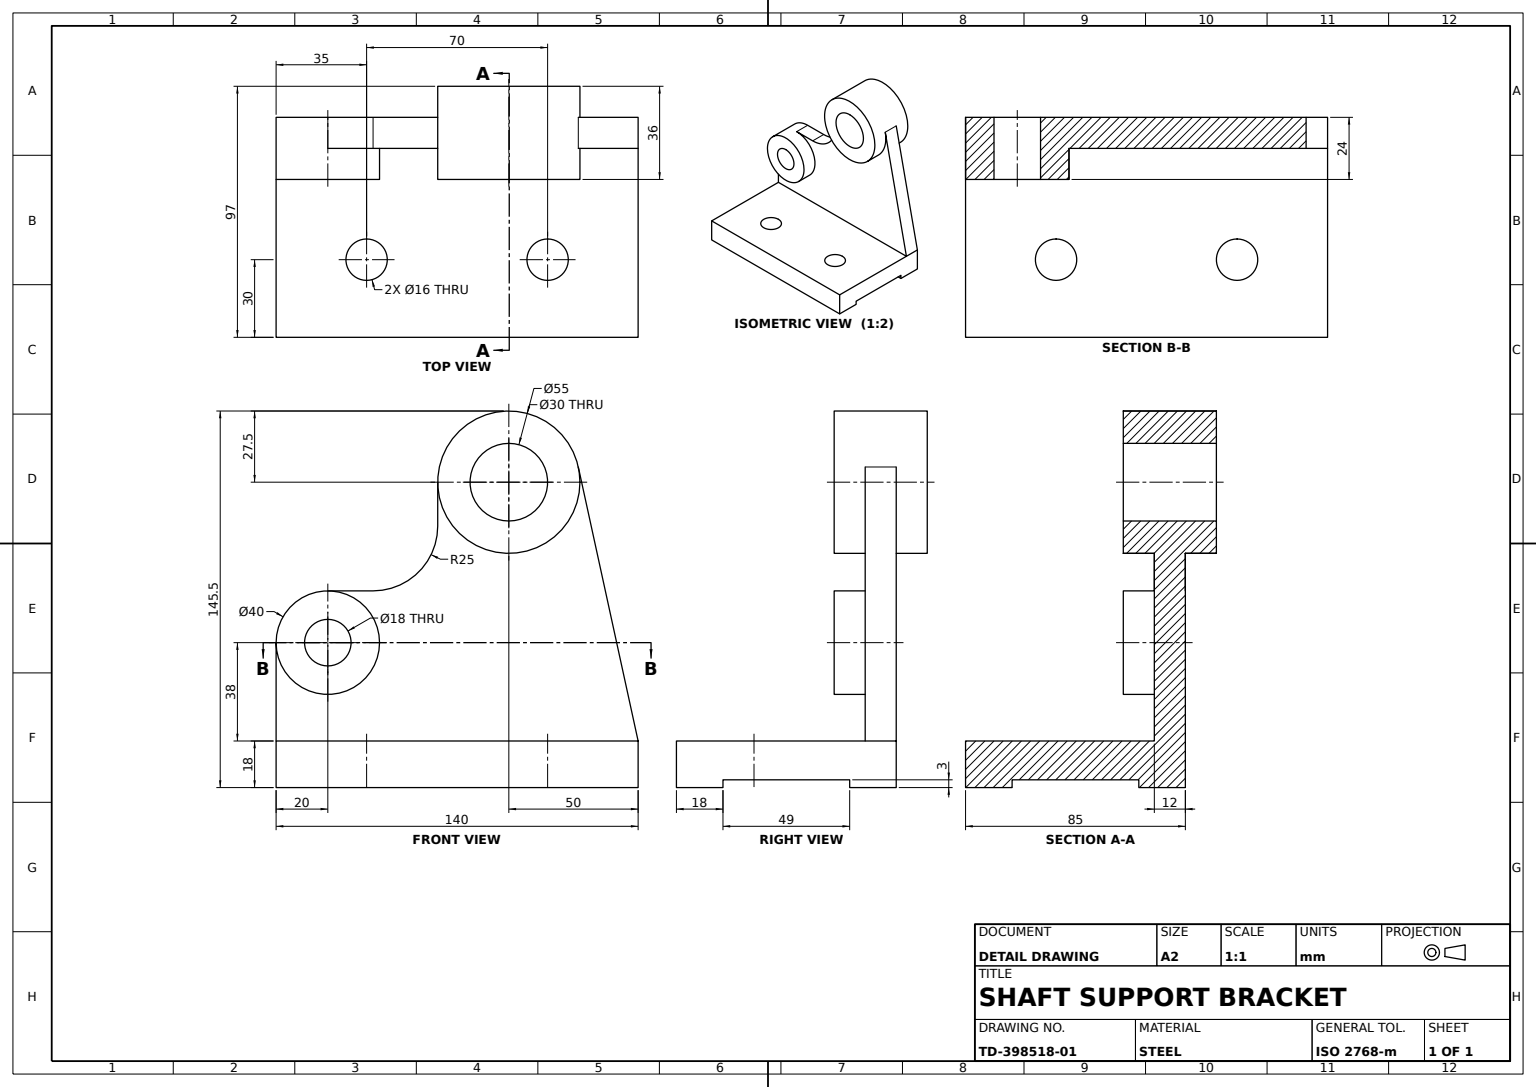
ISO-10303-21;
HEADER;
FILE_DESCRIPTION((''),'2;1');
FILE_NAME('','',(''),(''),'','','');
FILE_SCHEMA(('AUTOMOTIVE_DESIGN'));
ENDSEC;
DATA;
#1=APPLICATION_CONTEXT('');
#2=PRODUCT_CONTEXT('',#1,'mechanical');
#3=PRODUCT('','','',(#2));
#4=PRODUCT_DEFINITION_FORMATION('','',#3);
#5=PRODUCT_DEFINITION_CONTEXT('',#1,'design');
#6=PRODUCT_DEFINITION('','',#4,#5);
#7=PRODUCT_DEFINITION_SHAPE('','',#6);
#8=(LENGTH_UNIT()NAMED_UNIT(*)SI_UNIT(.MILLI.,.METRE.));
#9=(NAMED_UNIT(*)PLANE_ANGLE_UNIT()SI_UNIT($,.RADIAN.));
#10=(NAMED_UNIT(*)SI_UNIT($,.STERADIAN.)SOLID_ANGLE_UNIT());
#11=UNCERTAINTY_MEASURE_WITH_UNIT(LENGTH_MEASURE(0.005),#8,'distance_accuracy_value','');
#12=(GEOMETRIC_REPRESENTATION_CONTEXT(3)GLOBAL_UNCERTAINTY_ASSIGNED_CONTEXT((#11))GLOBAL_UNIT_ASSIGNED_CONTEXT((#8,#9,#10))REPRESENTATION_CONTEXT('',''));
#13=CARTESIAN_POINT('',(-18.5,-50.,65.));
#14=VERTEX_POINT('',#13);
#15=CARTESIAN_POINT('',(-18.5,-50.,56.));
#16=DIRECTION('',(-1.,0.,0.));
#17=DIRECTION('',(0.,0.,1.));
#18=AXIS2_PLACEMENT_3D('',#15,#16,#17);
#19=CIRCLE('',#18,9.);
#20=EDGE_CURVE('',#14,#14,#19,.T.);
#21=ORIENTED_EDGE('',*,*,#20,.T.);
#22=EDGE_LOOP('',(#21));
#23=FACE_BOUND('',#22,.T.);
#24=CARTESIAN_POINT('',(-18.5,-30.,56.));
#25=VERTEX_POINT('',#24);
#26=DIRECTION('',(1.,0.,0.));
#27=DIRECTION('',(0.,1.,0.));
#28=AXIS2_PLACEMENT_3D('',#15,#26,#27);
#29=CIRCLE('',#28,20.);
#30=EDGE_CURVE('',#25,#25,#29,.T.);
#31=ORIENTED_EDGE('',*,*,#30,.T.);
#32=EDGE_LOOP('',(#31));
#33=FACE_BOUND('',#32,.T.);
#34=DIRECTION('',(0.,0.,-1.));
#35=AXIS2_PLACEMENT_3D('',#15,#26,#34);
#36=PLANE('',#35);
#37=ADVANCED_FACE('',(#23,#33),#36,.T.);
#38=CARTESIAN_POINT('',(20.5,35.,3.));
#39=VERTEX_POINT('',#38);
#40=CARTESIAN_POINT('',(12.5,35.,3.));
#41=AXIS2_PLACEMENT_3D('',#40,#17,#26);
#42=CIRCLE('',#41,8.);
#43=EDGE_CURVE('',#39,#39,#42,.T.);
#44=ORIENTED_EDGE('',*,*,#43,.T.);
#45=EDGE_LOOP('',(#44));
#46=FACE_BOUND('',#45,.T.);
#47=CARTESIAN_POINT('',(20.5,-35.,3.));
#48=VERTEX_POINT('',#47);
#49=CARTESIAN_POINT('',(12.5,-35.,3.));
#50=AXIS2_PLACEMENT_3D('',#49,#17,#26);
#51=CIRCLE('',#50,8.);
#52=EDGE_CURVE('',#48,#48,#51,.T.);
#53=ORIENTED_EDGE('',*,*,#52,.T.);
#54=EDGE_LOOP('',(#53));
#55=FACE_BOUND('',#54,.T.);
#56=CARTESIAN_POINT('',(-24.5,-70.,3.));
#57=VERTEX_POINT('',#56);
#58=CARTESIAN_POINT('',(24.5,-70.,3.));
#59=VERTEX_POINT('',#58);
#60=CARTESIAN_POINT('',(0.,-70.,3.));
#61=VECTOR('',#26,1000.);
#62=LINE('',#60,#61);
#63=EDGE_CURVE('',#57,#59,#62,.T.);
#64=ORIENTED_EDGE('',*,*,#63,.F.);
#65=CARTESIAN_POINT('',(-24.5,70.,3.));
#66=VERTEX_POINT('',#65);
#67=CARTESIAN_POINT('',(-24.5,-78.,3.));
#68=VECTOR('',#27,1000.);
#69=LINE('',#67,#68);
#70=EDGE_CURVE('',#66,#57,#69,.F.);
#71=ORIENTED_EDGE('',*,*,#70,.F.);
#72=CARTESIAN_POINT('',(24.5,70.,3.));
#73=VERTEX_POINT('',#72);
#74=CARTESIAN_POINT('',(0.,70.,3.));
#75=LINE('',#74,#61);
#76=EDGE_CURVE('',#66,#73,#75,.T.);
#77=ORIENTED_EDGE('',*,*,#76,.T.);
#78=CARTESIAN_POINT('',(24.5,-78.,3.));
#79=LINE('',#78,#68);
#80=EDGE_CURVE('',#73,#59,#79,.F.);
#81=ORIENTED_EDGE('',*,*,#80,.T.);
#82=EDGE_LOOP('',(#64,#71,#77,#81));
#83=FACE_BOUND('',#82,.T.);
#84=AXIS2_PLACEMENT_3D('',#67,#17,#26);
#85=PLANE('',#84);
#86=ADVANCED_FACE('',(#46,#55,#83),#85,.F.);
#87=ORIENTED_EDGE('',*,*,#30,.F.);
#88=EDGE_LOOP('',(#87));
#89=FACE_BOUND('',#88,.T.);
#90=CARTESIAN_POINT('',(-42.5,-70.,56.));
#91=VERTEX_POINT('',#90);
#92=CARTESIAN_POINT('',(-30.5,-70.,56.));
#93=VERTEX_POINT('',#92);
#94=LINE('',#90,#61);
#95=EDGE_CURVE('',#91,#93,#94,.T.);
#96=ORIENTED_EDGE('',*,*,#95,.T.);
#97=CARTESIAN_POINT('',(-30.5,-50.,76.));
#98=VERTEX_POINT('',#97);
#99=CARTESIAN_POINT('',(-30.5,-50.,56.));
#100=AXIS2_PLACEMENT_3D('',#99,#16,#17);
#101=CIRCLE('',#100,20.);
#102=EDGE_CURVE('',#93,#98,#101,.F.);
#103=ORIENTED_EDGE('',*,*,#102,.T.);
#104=CARTESIAN_POINT('',(-42.5,-50.,76.));
#105=VERTEX_POINT('',#104);
#106=LINE('',#104,#61);
#107=EDGE_CURVE('',#105,#98,#106,.T.);
#108=ORIENTED_EDGE('',*,*,#107,.F.);
#109=CARTESIAN_POINT('',(-42.5,-50.,56.));
#110=AXIS2_PLACEMENT_3D('',#109,#16,#27);
#111=CIRCLE('',#110,20.);
#112=EDGE_CURVE('',#91,#105,#111,.T.);
#113=ORIENTED_EDGE('',*,*,#112,.F.);
#114=EDGE_LOOP('',(#96,#103,#108,#113));
#115=FACE_BOUND('',#114,.T.);
#116=AXIS2_PLACEMENT_3D('',#109,#26,#34);
#117=CYLINDRICAL_SURFACE('',#116,20.);
#118=ADVANCED_FACE('',(#89,#115),#117,.T.);
#119=CARTESIAN_POINT('',(4.5,35.,18.));
#120=VERTEX_POINT('',#119);
#121=CARTESIAN_POINT('',(12.5,35.,18.));
#122=AXIS2_PLACEMENT_3D('',#121,#34,#16);
#123=CIRCLE('',#122,8.);
#124=EDGE_CURVE('',#120,#120,#123,.T.);
#125=ORIENTED_EDGE('',*,*,#124,.T.);
#126=EDGE_LOOP('',(#125));
#127=FACE_BOUND('',#126,.T.);
#128=CARTESIAN_POINT('',(42.5,70.,18.));
#129=VERTEX_POINT('',#128);
#130=CARTESIAN_POINT('',(42.5,-70.,18.));
#131=VERTEX_POINT('',#130);
#132=DIRECTION('',(0.,-1.,0.));
#133=VECTOR('',#132,1000.);
#134=LINE('',#128,#133);
#135=EDGE_CURVE('',#129,#131,#134,.T.);
#136=ORIENTED_EDGE('',*,*,#135,.F.);
#137=CARTESIAN_POINT('',(-30.5,70.,18.));
#138=VERTEX_POINT('',#137);
#139=CARTESIAN_POINT('',(-42.5,70.,18.));
#140=LINE('',#139,#61);
#141=EDGE_CURVE('',#138,#129,#140,.T.);
#142=ORIENTED_EDGE('',*,*,#141,.F.);
#143=CARTESIAN_POINT('',(-30.5,-70.,18.));
#144=VERTEX_POINT('',#143);
#145=LINE('',#137,#133);
#146=EDGE_CURVE('',#138,#144,#145,.T.);
#147=ORIENTED_EDGE('',*,*,#146,.T.);
#148=CARTESIAN_POINT('',(-42.5,-70.,18.));
#149=LINE('',#148,#61);
#150=EDGE_CURVE('',#144,#131,#149,.T.);
#151=ORIENTED_EDGE('',*,*,#150,.T.);
#152=EDGE_LOOP('',(#136,#142,#147,#151));
#153=FACE_BOUND('',#152,.T.);
#154=CARTESIAN_POINT('',(4.5,-35.,18.));
#155=VERTEX_POINT('',#154);
#156=CARTESIAN_POINT('',(12.5,-35.,18.));
#157=AXIS2_PLACEMENT_3D('',#156,#34,#16);
#158=CIRCLE('',#157,8.);
#159=EDGE_CURVE('',#155,#155,#158,.T.);
#160=ORIENTED_EDGE('',*,*,#159,.T.);
#161=EDGE_LOOP('',(#160));
#162=FACE_BOUND('',#161,.T.);
#163=AXIS2_PLACEMENT_3D('',#139,#34,#16);
#164=PLANE('',#163);
#165=ADVANCED_FACE('',(#127,#153,#162),#164,.F.);
#166=CARTESIAN_POINT('',(42.5,70.,0.));
#167=VERTEX_POINT('',#166);
#168=CARTESIAN_POINT('',(24.5,70.,0.));
#169=VERTEX_POINT('',#168);
#170=VECTOR('',#16,1000.);
#171=LINE('',#166,#170);
#172=EDGE_CURVE('',#167,#169,#171,.T.);
#173=ORIENTED_EDGE('',*,*,#172,.F.);
#174=CARTESIAN_POINT('',(42.5,-70.,0.));
#175=VERTEX_POINT('',#174);
#176=LINE('',#166,#133);
#177=EDGE_CURVE('',#167,#175,#176,.T.);
#178=ORIENTED_EDGE('',*,*,#177,.T.);
#179=CARTESIAN_POINT('',(24.5,-70.,0.));
#180=VERTEX_POINT('',#179);
#181=LINE('',#174,#170);
#182=EDGE_CURVE('',#175,#180,#181,.T.);
#183=ORIENTED_EDGE('',*,*,#182,.T.);
#184=CARTESIAN_POINT('',(24.5,-78.,0.));
#185=LINE('',#184,#68);
#186=EDGE_CURVE('',#180,#169,#185,.T.);
#187=ORIENTED_EDGE('',*,*,#186,.T.);
#188=EDGE_LOOP('',(#173,#178,#183,#187));
#189=FACE_BOUND('',#188,.T.);
#190=AXIS2_PLACEMENT_3D('',#166,#17,#26);
#191=PLANE('',#190);
#192=ADVANCED_FACE('',(#189),#191,.F.);
#193=VECTOR('',#34,1000.);
#194=LINE('',#179,#193);
#195=EDGE_CURVE('',#59,#180,#194,.T.);
#196=ORIENTED_EDGE('',*,*,#195,.F.);
#197=ORIENTED_EDGE('',*,*,#80,.F.);
#198=LINE('',#168,#193);
#199=EDGE_CURVE('',#73,#169,#198,.T.);
#200=ORIENTED_EDGE('',*,*,#199,.T.);
#201=ORIENTED_EDGE('',*,*,#186,.F.);
#202=EDGE_LOOP('',(#196,#197,#200,#201));
#203=FACE_BOUND('',#202,.T.);
#204=AXIS2_PLACEMENT_3D('',#78,#26,#34);
#205=PLANE('',#204);
#206=ADVANCED_FACE('',(#203),#205,.F.);
#207=CARTESIAN_POINT('',(-42.5,-50.,47.));
#208=VERTEX_POINT('',#207);
#209=CIRCLE('',#116,9.);
#210=EDGE_CURVE('',#208,#208,#209,.T.);
#211=ORIENTED_EDGE('',*,*,#210,.T.);
#212=EDGE_LOOP('',(#211));
#213=FACE_BOUND('',#212,.T.);
#214=CARTESIAN_POINT('',(-42.5,70.,0.));
#215=VERTEX_POINT('',#214);
#216=CARTESIAN_POINT('',(-42.5,-70.,0.));
#217=VERTEX_POINT('',#216);
#218=LINE('',#214,#133);
#219=EDGE_CURVE('',#215,#217,#218,.T.);
#220=ORIENTED_EDGE('',*,*,#219,.T.);
#221=VECTOR('',#17,1000.);
#222=LINE('',#216,#221);
#223=EDGE_CURVE('',#217,#91,#222,.T.);
#224=ORIENTED_EDGE('',*,*,#223,.T.);
#225=ORIENTED_EDGE('',*,*,#112,.T.);
#226=CARTESIAN_POINT('',(-42.5,-32.5,76.));
#227=VERTEX_POINT('',#226);
#228=LINE('',#104,#68);
#229=EDGE_CURVE('',#105,#227,#228,.T.);
#230=ORIENTED_EDGE('',*,*,#229,.T.);
#231=CARTESIAN_POINT('',(-42.5,-7.5,101.));
#232=VERTEX_POINT('',#231);
#233=CARTESIAN_POINT('',(-42.5,-32.5,101.));
#234=AXIS2_PLACEMENT_3D('',#233,#26,#34);
#235=CIRCLE('',#234,25.);
#236=EDGE_CURVE('',#227,#232,#235,.T.);
#237=ORIENTED_EDGE('',*,*,#236,.T.);
#238=CARTESIAN_POINT('',(-42.5,-7.5,118.));
#239=VERTEX_POINT('',#238);
#240=CARTESIAN_POINT('',(-42.5,-7.5,76.));
#241=LINE('',#240,#221);
#242=EDGE_CURVE('',#232,#239,#241,.T.);
#243=ORIENTED_EDGE('',*,*,#242,.T.);
#244=CARTESIAN_POINT('',(-42.5,46.866088,123.870544));
#245=VERTEX_POINT('',#244);
#246=CARTESIAN_POINT('',(-42.5,20.,118.));
#247=AXIS2_PLACEMENT_3D('',#246,#26,#34);
#248=CIRCLE('',#247,27.5);
#249=EDGE_CURVE('',#239,#245,#248,.T.);
#250=ORIENTED_EDGE('',*,*,#249,.T.);
#251=VERTEX_POINT('',#139);
#252=DIRECTION('',(0.,0.213474336,-0.976948672));
#253=VECTOR('',#252,1000.);
#254=LINE('',#244,#253);
#255=EDGE_CURVE('',#245,#251,#254,.T.);
#256=ORIENTED_EDGE('',*,*,#255,.T.);
#257=LINE('',#214,#221);
#258=EDGE_CURVE('',#215,#251,#257,.T.);
#259=ORIENTED_EDGE('',*,*,#258,.F.);
#260=EDGE_LOOP('',(#220,#224,#225,#230,#237,#243,#250,#256,#259));
#261=FACE_BOUND('',#260,.T.);
#262=AXIS2_PLACEMENT_3D('',#214,#26,#34);
#263=PLANE('',#262);
#264=ADVANCED_FACE('',(#213,#261),#263,.F.);
#265=ORIENTED_EDGE('',*,*,#70,.T.);
#266=CARTESIAN_POINT('',(-24.5,-70.,0.));
#267=VERTEX_POINT('',#266);
#268=LINE('',#266,#221);
#269=EDGE_CURVE('',#267,#57,#268,.T.);
#270=ORIENTED_EDGE('',*,*,#269,.F.);
#271=CARTESIAN_POINT('',(-24.5,70.,0.));
#272=VERTEX_POINT('',#271);
#273=CARTESIAN_POINT('',(-24.5,-78.,0.));
#274=LINE('',#273,#68);
#275=EDGE_CURVE('',#267,#272,#274,.T.);
#276=ORIENTED_EDGE('',*,*,#275,.T.);
#277=LINE('',#271,#221);
#278=EDGE_CURVE('',#272,#66,#277,.T.);
#279=ORIENTED_EDGE('',*,*,#278,.T.);
#280=EDGE_LOOP('',(#265,#270,#276,#279));
#281=FACE_BOUND('',#280,.T.);
#282=AXIS2_PLACEMENT_3D('',#273,#16,#17);
#283=PLANE('',#282);
#284=ADVANCED_FACE('',(#281),#283,.F.);
#285=EDGE_CURVE('',#272,#215,#171,.T.);
#286=ORIENTED_EDGE('',*,*,#285,.F.);
#287=ORIENTED_EDGE('',*,*,#275,.F.);
#288=EDGE_CURVE('',#267,#217,#181,.T.);
#289=ORIENTED_EDGE('',*,*,#288,.T.);
#290=ORIENTED_EDGE('',*,*,#219,.F.);
#291=EDGE_LOOP('',(#286,#287,#289,#290));
#292=FACE_BOUND('',#291,.T.);
#293=ADVANCED_FACE('',(#292),#191,.F.);
#294=ORIENTED_EDGE('',*,*,#172,.T.);
#295=ORIENTED_EDGE('',*,*,#199,.F.);
#296=ORIENTED_EDGE('',*,*,#76,.F.);
#297=ORIENTED_EDGE('',*,*,#278,.F.);
#298=ORIENTED_EDGE('',*,*,#285,.T.);
#299=ORIENTED_EDGE('',*,*,#258,.T.);
#300=EDGE_CURVE('',#251,#138,#140,.T.);
#301=ORIENTED_EDGE('',*,*,#300,.T.);
#302=ORIENTED_EDGE('',*,*,#141,.T.);
#303=LINE('',#128,#193);
#304=EDGE_CURVE('',#129,#167,#303,.T.);
#305=ORIENTED_EDGE('',*,*,#304,.T.);
#306=EDGE_LOOP('',(#294,#295,#296,#297,#298,#299,#301,#302,#305));
#307=FACE_BOUND('',#306,.T.);
#308=CARTESIAN_POINT('',(0.,70.,0.));
#309=AXIS2_PLACEMENT_3D('',#308,#27,#17);
#310=PLANE('',#309);
#311=ADVANCED_FACE('',(#307),#310,.T.);
#312=CARTESIAN_POINT('',(-54.5,20.,103.));
#313=VERTEX_POINT('',#312);
#314=CARTESIAN_POINT('',(-54.5,20.,118.));
#315=AXIS2_PLACEMENT_3D('',#314,#26,#34);
#316=CIRCLE('',#315,15.);
#317=EDGE_CURVE('',#313,#313,#316,.T.);
#318=ORIENTED_EDGE('',*,*,#317,.T.);
#319=EDGE_LOOP('',(#318));
#320=FACE_BOUND('',#319,.T.);
#321=CARTESIAN_POINT('',(-54.5,47.5,118.));
#322=VERTEX_POINT('',#321);
#323=AXIS2_PLACEMENT_3D('',#314,#26,#27);
#324=CIRCLE('',#323,27.5);
#325=EDGE_CURVE('',#322,#322,#324,.T.);
#326=ORIENTED_EDGE('',*,*,#325,.F.);
#327=EDGE_LOOP('',(#326));
#328=FACE_BOUND('',#327,.T.);
#329=PLANE('',#315);
#330=ADVANCED_FACE('',(#320,#328),#329,.F.);
#331=ORIENTED_EDGE('',*,*,#52,.F.);
#332=EDGE_LOOP('',(#331));
#333=FACE_BOUND('',#332,.T.);
#334=ORIENTED_EDGE('',*,*,#159,.F.);
#335=EDGE_LOOP('',(#334));
#336=FACE_BOUND('',#335,.T.);
#337=CYLINDRICAL_SURFACE('',#157,8.);
#338=ADVANCED_FACE('',(#333,#336),#337,.F.);
#339=ORIENTED_EDGE('',*,*,#146,.F.);
#340=CARTESIAN_POINT('',(-30.5,46.866088,123.870544));
#341=VERTEX_POINT('',#340);
#342=LINE('',#340,#253);
#343=EDGE_CURVE('',#341,#138,#342,.T.);
#344=ORIENTED_EDGE('',*,*,#343,.F.);
#345=CARTESIAN_POINT('',(-30.5,-7.5,118.));
#346=VERTEX_POINT('',#345);
#347=CARTESIAN_POINT('',(-30.5,20.,118.));
#348=AXIS2_PLACEMENT_3D('',#347,#16,#17);
#349=CIRCLE('',#348,27.5);
#350=EDGE_CURVE('',#346,#341,#349,.F.);
#351=ORIENTED_EDGE('',*,*,#350,.F.);
#352=CARTESIAN_POINT('',(-30.5,-7.5,101.));
#353=VERTEX_POINT('',#352);
#354=CARTESIAN_POINT('',(-30.5,-7.5,76.));
#355=LINE('',#354,#221);
#356=EDGE_CURVE('',#353,#346,#355,.T.);
#357=ORIENTED_EDGE('',*,*,#356,.F.);
#358=CARTESIAN_POINT('',(-30.5,-32.5,76.));
#359=VERTEX_POINT('',#358);
#360=CARTESIAN_POINT('',(-30.5,-32.5,101.));
#361=AXIS2_PLACEMENT_3D('',#360,#16,#17);
#362=CIRCLE('',#361,25.);
#363=EDGE_CURVE('',#353,#359,#362,.T.);
#364=ORIENTED_EDGE('',*,*,#363,.T.);
#365=LINE('',#97,#68);
#366=EDGE_CURVE('',#98,#359,#365,.T.);
#367=ORIENTED_EDGE('',*,*,#366,.F.);
#368=ORIENTED_EDGE('',*,*,#102,.F.);
#369=LINE('',#143,#221);
#370=EDGE_CURVE('',#144,#93,#369,.T.);
#371=ORIENTED_EDGE('',*,*,#370,.F.);
#372=EDGE_LOOP('',(#339,#344,#351,#357,#364,#367,#368,#371));
#373=FACE_BOUND('',#372,.T.);
#374=PLANE('',#348);
#375=ADVANCED_FACE('',(#373),#374,.F.);
#376=ORIENTED_EDGE('',*,*,#229,.F.);
#377=ORIENTED_EDGE('',*,*,#107,.T.);
#378=ORIENTED_EDGE('',*,*,#366,.T.);
#379=LINE('',#226,#61);
#380=EDGE_CURVE('',#359,#227,#379,.F.);
#381=ORIENTED_EDGE('',*,*,#380,.T.);
#382=EDGE_LOOP('',(#376,#377,#378,#381));
#383=FACE_BOUND('',#382,.T.);
#384=AXIS2_PLACEMENT_3D('',#104,#34,#16);
#385=PLANE('',#384);
#386=ADVANCED_FACE('',(#383),#385,.F.);
#387=ORIENTED_EDGE('',*,*,#343,.T.);
#388=ORIENTED_EDGE('',*,*,#300,.F.);
#389=ORIENTED_EDGE('',*,*,#255,.F.);
#390=LINE('',#244,#61);
#391=EDGE_CURVE('',#245,#341,#390,.T.);
#392=ORIENTED_EDGE('',*,*,#391,.T.);
#393=EDGE_LOOP('',(#387,#388,#389,#392));
#394=FACE_BOUND('',#393,.T.);
#395=DIRECTION('',(0.,-0.976948672,-0.213474336));
#396=AXIS2_PLACEMENT_3D('',#244,#395,#252);
#397=PLANE('',#396);
#398=ADVANCED_FACE('',(#394),#397,.F.);
#399=CARTESIAN_POINT('',(-18.5,20.,133.));
#400=VERTEX_POINT('',#399);
#401=CARTESIAN_POINT('',(-18.5,20.,118.));
#402=AXIS2_PLACEMENT_3D('',#401,#16,#17);
#403=CIRCLE('',#402,15.);
#404=EDGE_CURVE('',#400,#400,#403,.T.);
#405=ORIENTED_EDGE('',*,*,#404,.T.);
#406=EDGE_LOOP('',(#405));
#407=FACE_BOUND('',#406,.T.);
#408=CARTESIAN_POINT('',(-18.5,47.5,118.));
#409=VERTEX_POINT('',#408);
#410=AXIS2_PLACEMENT_3D('',#401,#26,#27);
#411=CIRCLE('',#410,27.5);
#412=EDGE_CURVE('',#409,#409,#411,.T.);
#413=ORIENTED_EDGE('',*,*,#412,.T.);
#414=EDGE_LOOP('',(#413));
#415=FACE_BOUND('',#414,.T.);
#416=AXIS2_PLACEMENT_3D('',#401,#26,#34);
#417=PLANE('',#416);
#418=ADVANCED_FACE('',(#407,#415),#417,.T.);
#419=ORIENTED_EDGE('',*,*,#210,.F.);
#420=EDGE_LOOP('',(#419));
#421=FACE_BOUND('',#420,.T.);
#422=ORIENTED_EDGE('',*,*,#20,.F.);
#423=EDGE_LOOP('',(#422));
#424=FACE_BOUND('',#423,.T.);
#425=CYLINDRICAL_SURFACE('',#18,9.);
#426=ADVANCED_FACE('',(#421,#424),#425,.F.);
#427=ORIENTED_EDGE('',*,*,#43,.F.);
#428=EDGE_LOOP('',(#427));
#429=FACE_BOUND('',#428,.T.);
#430=ORIENTED_EDGE('',*,*,#124,.F.);
#431=EDGE_LOOP('',(#430));
#432=FACE_BOUND('',#431,.T.);
#433=CYLINDRICAL_SURFACE('',#122,8.);
#434=ADVANCED_FACE('',(#429,#432),#433,.F.);
#435=ORIENTED_EDGE('',*,*,#404,.F.);
#436=EDGE_LOOP('',(#435));
#437=FACE_BOUND('',#436,.T.);
#438=ORIENTED_EDGE('',*,*,#317,.F.);
#439=EDGE_LOOP('',(#438));
#440=FACE_BOUND('',#439,.T.);
#441=CYLINDRICAL_SURFACE('',#402,15.);
#442=ADVANCED_FACE('',(#437,#440),#441,.F.);
#443=ORIENTED_EDGE('',*,*,#135,.T.);
#444=LINE('',#130,#193);
#445=EDGE_CURVE('',#131,#175,#444,.T.);
#446=ORIENTED_EDGE('',*,*,#445,.T.);
#447=ORIENTED_EDGE('',*,*,#177,.F.);
#448=ORIENTED_EDGE('',*,*,#304,.F.);
#449=EDGE_LOOP('',(#443,#446,#447,#448));
#450=FACE_BOUND('',#449,.T.);
#451=AXIS2_PLACEMENT_3D('',#128,#16,#17);
#452=PLANE('',#451);
#453=ADVANCED_FACE('',(#450),#452,.F.);
#454=ORIENTED_EDGE('',*,*,#350,.T.);
#455=ORIENTED_EDGE('',*,*,#391,.F.);
#456=ORIENTED_EDGE('',*,*,#249,.F.);
#457=LINE('',#238,#61);
#458=EDGE_CURVE('',#239,#346,#457,.T.);
#459=ORIENTED_EDGE('',*,*,#458,.T.);
#460=EDGE_LOOP('',(#454,#455,#456,#459));
#461=FACE_BOUND('',#460,.T.);
#462=ORIENTED_EDGE('',*,*,#412,.F.);
#463=EDGE_LOOP('',(#462));
#464=FACE_BOUND('',#463,.T.);
#465=ORIENTED_EDGE('',*,*,#325,.T.);
#466=EDGE_LOOP('',(#465));
#467=FACE_BOUND('',#466,.T.);
#468=CYLINDRICAL_SURFACE('',#247,27.5);
#469=ADVANCED_FACE('',(#461,#464,#467),#468,.T.);
#470=ORIENTED_EDGE('',*,*,#380,.F.);
#471=ORIENTED_EDGE('',*,*,#363,.F.);
#472=LINE('',#352,#61);
#473=EDGE_CURVE('',#232,#353,#472,.T.);
#474=ORIENTED_EDGE('',*,*,#473,.F.);
#475=ORIENTED_EDGE('',*,*,#236,.F.);
#476=EDGE_LOOP('',(#470,#471,#474,#475));
#477=FACE_BOUND('',#476,.T.);
#478=AXIS2_PLACEMENT_3D('',#233,#16,#17);
#479=CYLINDRICAL_SURFACE('',#478,25.);
#480=ADVANCED_FACE('',(#477),#479,.F.);
#481=ORIENTED_EDGE('',*,*,#195,.T.);
#482=ORIENTED_EDGE('',*,*,#182,.F.);
#483=ORIENTED_EDGE('',*,*,#445,.F.);
#484=ORIENTED_EDGE('',*,*,#150,.F.);
#485=ORIENTED_EDGE('',*,*,#370,.T.);
#486=ORIENTED_EDGE('',*,*,#95,.F.);
#487=ORIENTED_EDGE('',*,*,#223,.F.);
#488=ORIENTED_EDGE('',*,*,#288,.F.);
#489=ORIENTED_EDGE('',*,*,#269,.T.);
#490=ORIENTED_EDGE('',*,*,#63,.T.);
#491=EDGE_LOOP('',(#481,#482,#483,#484,#485,#486,#487,#488,#489,#490));
#492=FACE_BOUND('',#491,.T.);
#493=CARTESIAN_POINT('',(0.,-70.,0.));
#494=AXIS2_PLACEMENT_3D('',#493,#27,#17);
#495=PLANE('',#494);
#496=ADVANCED_FACE('',(#492),#495,.F.);
#497=ORIENTED_EDGE('',*,*,#473,.T.);
#498=ORIENTED_EDGE('',*,*,#356,.T.);
#499=ORIENTED_EDGE('',*,*,#458,.F.);
#500=ORIENTED_EDGE('',*,*,#242,.F.);
#501=EDGE_LOOP('',(#497,#498,#499,#500));
#502=FACE_BOUND('',#501,.T.);
#503=AXIS2_PLACEMENT_3D('',#240,#27,#17);
#504=PLANE('',#503);
#505=ADVANCED_FACE('',(#502),#504,.F.);
#506=CLOSED_SHELL('',(#37,#86,#118,#165,#192,#206,#264,#284,#293,#311,#330,#338,#375,#386,#398,#418,#426,#434,#442,#453,#469,#480,#496,#505));
#507=MANIFOLD_SOLID_BREP('',#506);
#508=ADVANCED_BREP_SHAPE_REPRESENTATION('',(#507),#12);
#509=SHAPE_DEFINITION_REPRESENTATION(#7,#508);
ENDSEC;
END-ISO-10303-21;
